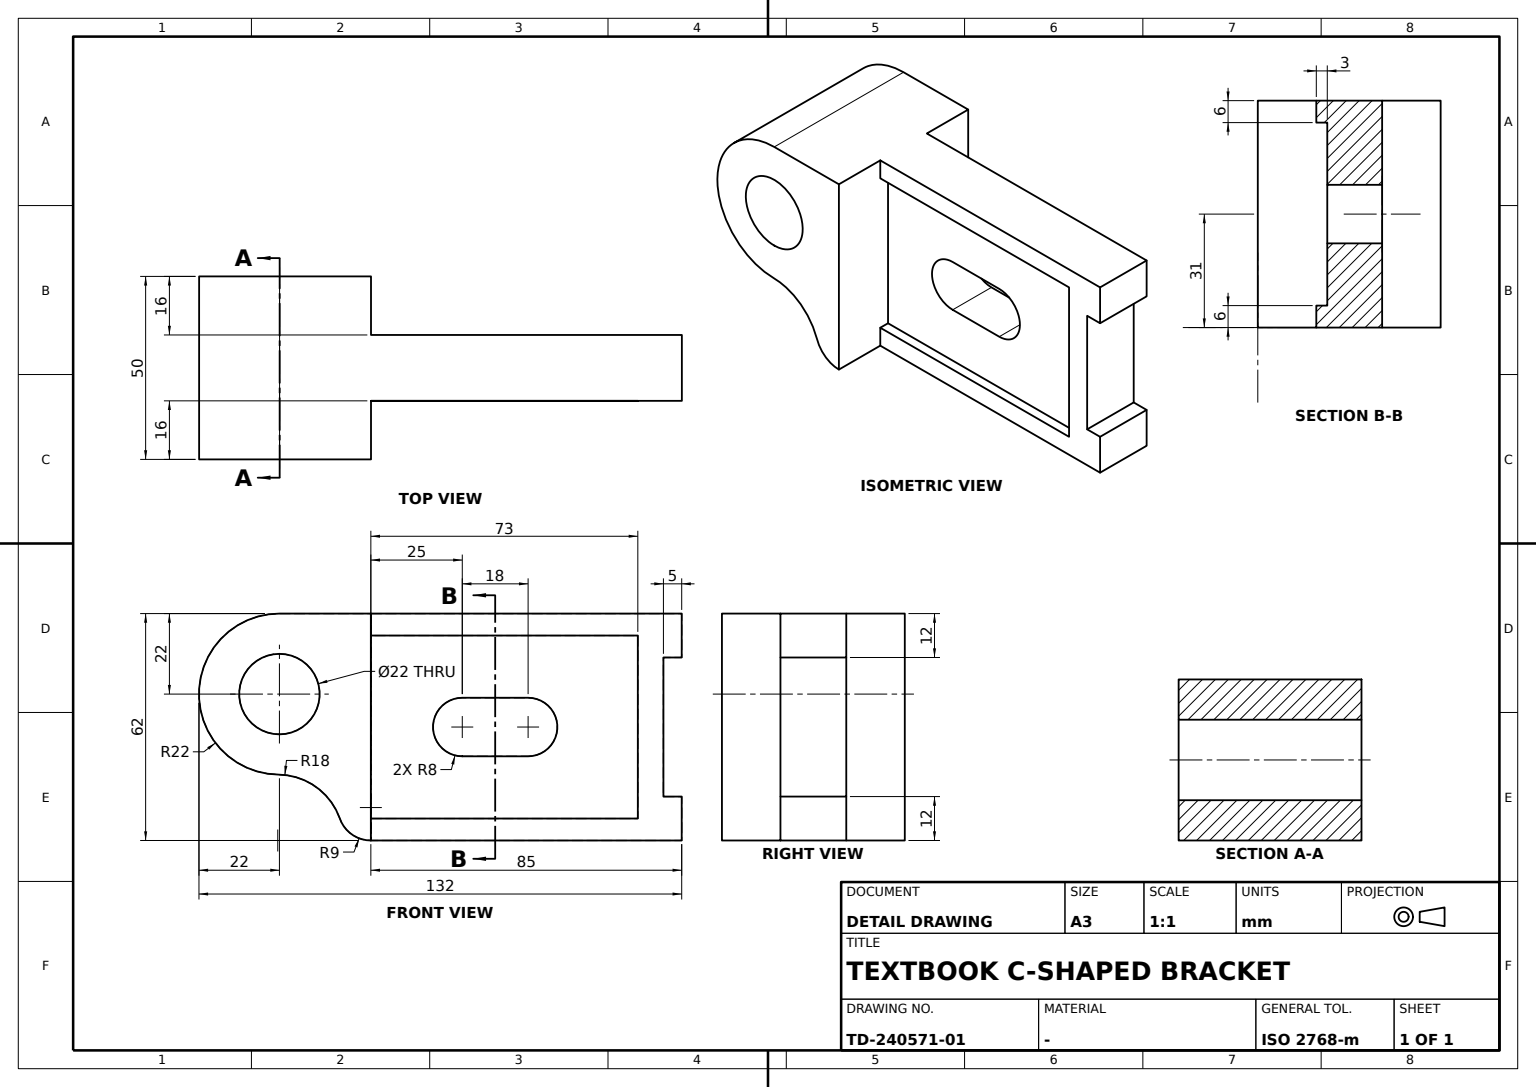
ISO-10303-21;
HEADER;
FILE_DESCRIPTION((''),'2;1');
FILE_NAME('','',(''),(''),'','','');
FILE_SCHEMA(('AUTOMOTIVE_DESIGN'));
ENDSEC;
DATA;
#1=APPLICATION_CONTEXT('');
#2=PRODUCT_CONTEXT('',#1,'mechanical');
#3=PRODUCT('','','',(#2));
#4=PRODUCT_DEFINITION_FORMATION('','',#3);
#5=PRODUCT_DEFINITION_CONTEXT('',#1,'design');
#6=PRODUCT_DEFINITION('','',#4,#5);
#7=PRODUCT_DEFINITION_SHAPE('','',#6);
#8=(LENGTH_UNIT()NAMED_UNIT(*)SI_UNIT(.MILLI.,.METRE.));
#9=(NAMED_UNIT(*)PLANE_ANGLE_UNIT()SI_UNIT($,.RADIAN.));
#10=(NAMED_UNIT(*)SI_UNIT($,.STERADIAN.)SOLID_ANGLE_UNIT());
#11=UNCERTAINTY_MEASURE_WITH_UNIT(LENGTH_MEASURE(0.005),#8,'distance_accuracy_value','');
#12=(GEOMETRIC_REPRESENTATION_CONTEXT(3)GLOBAL_UNCERTAINTY_ASSIGNED_CONTEXT((#11))GLOBAL_UNIT_ASSIGNED_CONTEXT((#8,#9,#10))REPRESENTATION_CONTEXT('',''));
#13=CARTESIAN_POINT('',(-9.,0.,-31.));
#14=VERTEX_POINT('',#13);
#15=CARTESIAN_POINT('',(-9.,0.,31.));
#16=VERTEX_POINT('',#15);
#17=CARTESIAN_POINT('',(-9.,0.,0.));
#18=DIRECTION('',(0.,0.,1.));
#19=VECTOR('',#18,1000.);
#20=LINE('',#17,#19);
#21=EDGE_CURVE('',#14,#16,#20,.T.);
#22=ORIENTED_EDGE('',*,*,#21,.F.);
#23=CARTESIAN_POINT('',(-25.,0.,-31.));
#24=VERTEX_POINT('',#23);
#25=DIRECTION('',(1.,0.,0.));
#26=VECTOR('',#25,1000.);
#27=LINE('',#23,#26);
#28=EDGE_CURVE('',#24,#14,#27,.T.);
#29=ORIENTED_EDGE('',*,*,#28,.F.);
#30=CARTESIAN_POINT('',(-25.,0.,31.));
#31=VERTEX_POINT('',#30);
#32=DIRECTION('',(0.,0.,-1.));
#33=VECTOR('',#32,1000.);
#34=LINE('',#23,#33);
#35=EDGE_CURVE('',#31,#24,#34,.T.);
#36=ORIENTED_EDGE('',*,*,#35,.F.);
#37=CARTESIAN_POINT('',(0.,0.,31.));
#38=LINE('',#37,#26);
#39=EDGE_CURVE('',#31,#16,#38,.T.);
#40=ORIENTED_EDGE('',*,*,#39,.T.);
#41=EDGE_LOOP('',(#22,#29,#36,#40));
#42=FACE_BOUND('',#41,.T.);
#43=CARTESIAN_POINT('',(0.,0.,-31.));
#44=DIRECTION('',(0.,1.,0.));
#45=AXIS2_PLACEMENT_3D('',#43,#44,#18);
#46=PLANE('',#45);
#47=ADVANCED_FACE('',(#42),#46,.T.);
#48=CARTESIAN_POINT('',(-25.,-25.,-2.));
#49=VERTEX_POINT('',#48);
#50=CARTESIAN_POINT('',(-25.,-25.,9.));
#51=AXIS2_PLACEMENT_3D('',#50,#25,#32);
#52=CIRCLE('',#51,11.);
#53=EDGE_CURVE('',#49,#49,#52,.T.);
#54=ORIENTED_EDGE('',*,*,#53,.F.);
#55=EDGE_LOOP('',(#54));
#56=FACE_BOUND('',#55,.T.);
#57=CARTESIAN_POINT('',(25.,-25.,-2.));
#58=VERTEX_POINT('',#57);
#59=CARTESIAN_POINT('',(25.,-25.,9.));
#60=AXIS2_PLACEMENT_3D('',#59,#25,#32);
#61=CIRCLE('',#60,11.);
#62=EDGE_CURVE('',#58,#58,#61,.T.);
#63=ORIENTED_EDGE('',*,*,#62,.T.);
#64=EDGE_LOOP('',(#63));
#65=FACE_BOUND('',#64,.T.);
#66=CARTESIAN_POINT('',(0.,-25.,9.));
#67=AXIS2_PLACEMENT_3D('',#66,#25,#44);
#68=CYLINDRICAL_SURFACE('',#67,11.);
#69=ADVANCED_FACE('',(#56,#65),#68,.F.);
#70=CARTESIAN_POINT('',(25.,-8.537319,-24.84854));
#71=VERTEX_POINT('',#70);
#72=CARTESIAN_POINT('',(25.,0.,-31.));
#73=VERTEX_POINT('',#72);
#74=CARTESIAN_POINT('',(25.,0.,-22.));
#75=AXIS2_PLACEMENT_3D('',#74,#25,#32);
#76=CIRCLE('',#75,9.);
#77=EDGE_CURVE('',#71,#73,#76,.T.);
#78=ORIENTED_EDGE('',*,*,#77,.T.);
#79=CARTESIAN_POINT('',(25.,0.,31.));
#80=VERTEX_POINT('',#79);
#81=LINE('',#72,#33);
#82=EDGE_CURVE('',#80,#73,#81,.T.);
#83=ORIENTED_EDGE('',*,*,#82,.F.);
#84=CARTESIAN_POINT('',(25.,-25.,31.));
#85=VERTEX_POINT('',#84);
#86=VECTOR('',#44,1000.);
#87=LINE('',#79,#86);
#88=EDGE_CURVE('',#85,#80,#87,.T.);
#89=ORIENTED_EDGE('',*,*,#88,.F.);
#90=CARTESIAN_POINT('',(25.,-25.24998,-12.99858));
#91=VERTEX_POINT('',#90);
#92=CIRCLE('',#60,22.);
#93=EDGE_CURVE('',#85,#91,#92,.T.);
#94=ORIENTED_EDGE('',*,*,#93,.T.);
#95=CARTESIAN_POINT('',(25.,-25.454509,-30.997418));
#96=AXIS2_PLACEMENT_3D('',#95,#25,#32);
#97=CIRCLE('',#96,18.);
#98=EDGE_CURVE('',#71,#91,#97,.T.);
#99=ORIENTED_EDGE('',*,*,#98,.F.);
#100=EDGE_LOOP('',(#78,#83,#89,#94,#99));
#101=FACE_BOUND('',#100,.T.);
#102=ORIENTED_EDGE('',*,*,#62,.F.);
#103=EDGE_LOOP('',(#102));
#104=FACE_BOUND('',#103,.T.);
#105=CARTESIAN_POINT('',(25.,0.,0.));
#106=AXIS2_PLACEMENT_3D('',#105,#25,#44);
#107=PLANE('',#106);
#108=ADVANCED_FACE('',(#101,#104),#107,.T.);
#109=CARTESIAN_POINT('',(6.,25.,-8.));
#110=VERTEX_POINT('',#109);
#111=CARTESIAN_POINT('',(6.,43.,-8.));
#112=VERTEX_POINT('',#111);
#113=LINE('',#109,#86);
#114=EDGE_CURVE('',#110,#112,#113,.T.);
#115=ORIENTED_EDGE('',*,*,#114,.T.);
#116=CARTESIAN_POINT('',(-9.,43.,-8.));
#117=VERTEX_POINT('',#116);
#118=CARTESIAN_POINT('',(-2.16,43.,-8.));
#119=LINE('',#118,#26);
#120=EDGE_CURVE('',#112,#117,#119,.F.);
#121=ORIENTED_EDGE('',*,*,#120,.T.);
#122=CARTESIAN_POINT('',(-9.,25.,-8.));
#123=VERTEX_POINT('',#122);
#124=LINE('',#122,#86);
#125=EDGE_CURVE('',#123,#117,#124,.T.);
#126=ORIENTED_EDGE('',*,*,#125,.F.);
#127=CARTESIAN_POINT('',(-2.16,25.,-8.));
#128=LINE('',#127,#26);
#129=EDGE_CURVE('',#110,#123,#128,.F.);
#130=ORIENTED_EDGE('',*,*,#129,.F.);
#131=EDGE_LOOP('',(#115,#121,#126,#130));
#132=FACE_BOUND('',#131,.T.);
#133=AXIS2_PLACEMENT_3D('',#109,#18,#44);
#134=PLANE('',#133);
#135=ADVANCED_FACE('',(#132),#134,.T.);
#136=CARTESIAN_POINT('',(6.,73.,25.));
#137=VERTEX_POINT('',#136);
#138=CARTESIAN_POINT('',(6.,73.,-25.));
#139=VERTEX_POINT('',#138);
#140=LINE('',#136,#33);
#141=EDGE_CURVE('',#137,#139,#140,.T.);
#142=ORIENTED_EDGE('',*,*,#141,.T.);
#143=CARTESIAN_POINT('',(9.,73.,-25.));
#144=VERTEX_POINT('',#143);
#145=DIRECTION('',(-1.,0.,0.));
#146=VECTOR('',#145,1000.);
#147=LINE('',#143,#146);
#148=EDGE_CURVE('',#144,#139,#147,.T.);
#149=ORIENTED_EDGE('',*,*,#148,.F.);
#150=CARTESIAN_POINT('',(9.,73.,25.));
#151=VERTEX_POINT('',#150);
#152=LINE('',#150,#33);
#153=EDGE_CURVE('',#151,#144,#152,.T.);
#154=ORIENTED_EDGE('',*,*,#153,.F.);
#155=LINE('',#150,#146);
#156=EDGE_CURVE('',#151,#137,#155,.T.);
#157=ORIENTED_EDGE('',*,*,#156,.T.);
#158=EDGE_LOOP('',(#142,#149,#154,#157));
#159=FACE_BOUND('',#158,.T.);
#160=AXIS2_PLACEMENT_3D('',#150,#44,#32);
#161=PLANE('',#160);
#162=ADVANCED_FACE('',(#159),#161,.F.);
#163=ORIENTED_EDGE('',*,*,#53,.T.);
#164=EDGE_LOOP('',(#163));
#165=FACE_BOUND('',#164,.T.);
#166=CARTESIAN_POINT('',(-25.,-8.537319,-24.84854));
#167=VERTEX_POINT('',#166);
#168=CARTESIAN_POINT('',(-25.,-25.24998,-12.99858));
#169=VERTEX_POINT('',#168);
#170=CARTESIAN_POINT('',(-25.,-25.454509,-30.997418));
#171=AXIS2_PLACEMENT_3D('',#170,#25,#32);
#172=CIRCLE('',#171,18.);
#173=EDGE_CURVE('',#167,#169,#172,.T.);
#174=ORIENTED_EDGE('',*,*,#173,.T.);
#175=CARTESIAN_POINT('',(-25.,-25.,31.));
#176=VERTEX_POINT('',#175);
#177=CIRCLE('',#51,22.);
#178=EDGE_CURVE('',#176,#169,#177,.T.);
#179=ORIENTED_EDGE('',*,*,#178,.F.);
#180=LINE('',#30,#86);
#181=EDGE_CURVE('',#176,#31,#180,.T.);
#182=ORIENTED_EDGE('',*,*,#181,.T.);
#183=ORIENTED_EDGE('',*,*,#35,.T.);
#184=CARTESIAN_POINT('',(-25.,0.,-22.));
#185=AXIS2_PLACEMENT_3D('',#184,#25,#32);
#186=CIRCLE('',#185,9.);
#187=EDGE_CURVE('',#167,#24,#186,.T.);
#188=ORIENTED_EDGE('',*,*,#187,.F.);
#189=EDGE_LOOP('',(#174,#179,#182,#183,#188));
#190=FACE_BOUND('',#189,.T.);
#191=CARTESIAN_POINT('',(-25.,0.,0.));
#192=AXIS2_PLACEMENT_3D('',#191,#25,#44);
#193=PLANE('',#192);
#194=ADVANCED_FACE('',(#165,#190),#193,.F.);
#195=LINE('',#166,#26);
#196=EDGE_CURVE('',#167,#71,#195,.T.);
#197=ORIENTED_EDGE('',*,*,#196,.T.);
#198=ORIENTED_EDGE('',*,*,#98,.T.);
#199=CARTESIAN_POINT('',(0.,-25.24998,-12.99858));
#200=LINE('',#199,#26);
#201=EDGE_CURVE('',#169,#91,#200,.T.);
#202=ORIENTED_EDGE('',*,*,#201,.F.);
#203=ORIENTED_EDGE('',*,*,#173,.F.);
#204=EDGE_LOOP('',(#197,#198,#202,#203));
#205=FACE_BOUND('',#204,.T.);
#206=CARTESIAN_POINT('',(0.,-25.454509,-30.997418));
#207=AXIS2_PLACEMENT_3D('',#206,#25,#44);
#208=CYLINDRICAL_SURFACE('',#207,18.);
#209=ADVANCED_FACE('',(#205),#208,.F.);
#210=CARTESIAN_POINT('',(6.,43.,8.));
#211=VERTEX_POINT('',#210);
#212=CARTESIAN_POINT('',(-9.,43.,8.));
#213=VERTEX_POINT('',#212);
#214=CARTESIAN_POINT('',(-2.16,43.,8.));
#215=LINE('',#214,#26);
#216=EDGE_CURVE('',#211,#213,#215,.F.);
#217=ORIENTED_EDGE('',*,*,#216,.T.);
#218=CARTESIAN_POINT('',(-9.,43.,0.));
#219=AXIS2_PLACEMENT_3D('',#218,#25,#32);
#220=CIRCLE('',#219,8.);
#221=EDGE_CURVE('',#117,#213,#220,.T.);
#222=ORIENTED_EDGE('',*,*,#221,.F.);
#223=ORIENTED_EDGE('',*,*,#120,.F.);
#224=CARTESIAN_POINT('',(6.,43.,0.));
#225=AXIS2_PLACEMENT_3D('',#224,#25,#32);
#226=CIRCLE('',#225,8.);
#227=EDGE_CURVE('',#112,#211,#226,.T.);
#228=ORIENTED_EDGE('',*,*,#227,.T.);
#229=EDGE_LOOP('',(#217,#222,#223,#228));
#230=FACE_BOUND('',#229,.T.);
#231=CARTESIAN_POINT('',(-2.16,43.,0.));
#232=AXIS2_PLACEMENT_3D('',#231,#25,#44);
#233=CYLINDRICAL_SURFACE('',#232,8.);
#234=ADVANCED_FACE('',(#230),#233,.F.);
#235=CARTESIAN_POINT('',(6.,25.,8.));
#236=VERTEX_POINT('',#235);
#237=CARTESIAN_POINT('',(-9.,25.,8.));
#238=VERTEX_POINT('',#237);
#239=CARTESIAN_POINT('',(-2.16,25.,8.));
#240=LINE('',#239,#26);
#241=EDGE_CURVE('',#236,#238,#240,.F.);
#242=ORIENTED_EDGE('',*,*,#241,.T.);
#243=LINE('',#237,#86);
#244=EDGE_CURVE('',#238,#213,#243,.T.);
#245=ORIENTED_EDGE('',*,*,#244,.T.);
#246=ORIENTED_EDGE('',*,*,#216,.F.);
#247=LINE('',#235,#86);
#248=EDGE_CURVE('',#236,#211,#247,.T.);
#249=ORIENTED_EDGE('',*,*,#248,.F.);
#250=EDGE_LOOP('',(#242,#245,#246,#249));
#251=FACE_BOUND('',#250,.T.);
#252=AXIS2_PLACEMENT_3D('',#235,#18,#44);
#253=PLANE('',#252);
#254=ADVANCED_FACE('',(#251),#253,.F.);
#255=CARTESIAN_POINT('',(-9.,80.,-19.));
#256=VERTEX_POINT('',#255);
#257=CARTESIAN_POINT('',(9.,80.,-19.));
#258=VERTEX_POINT('',#257);
#259=CARTESIAN_POINT('',(0.,80.,-19.));
#260=LINE('',#259,#26);
#261=EDGE_CURVE('',#256,#258,#260,.T.);
#262=ORIENTED_EDGE('',*,*,#261,.T.);
#263=CARTESIAN_POINT('',(9.,85.,-19.));
#264=VERTEX_POINT('',#263);
#265=CARTESIAN_POINT('',(9.,0.,-19.));
#266=LINE('',#265,#86);
#267=EDGE_CURVE('',#258,#264,#266,.T.);
#268=ORIENTED_EDGE('',*,*,#267,.T.);
#269=CARTESIAN_POINT('',(-9.,85.,-19.));
#270=VERTEX_POINT('',#269);
#271=CARTESIAN_POINT('',(0.,85.,-19.));
#272=LINE('',#271,#26);
#273=EDGE_CURVE('',#270,#264,#272,.T.);
#274=ORIENTED_EDGE('',*,*,#273,.F.);
#275=CARTESIAN_POINT('',(-9.,0.,-19.));
#276=LINE('',#275,#86);
#277=EDGE_CURVE('',#256,#270,#276,.T.);
#278=ORIENTED_EDGE('',*,*,#277,.F.);
#279=EDGE_LOOP('',(#262,#268,#274,#278));
#280=FACE_BOUND('',#279,.T.);
#281=AXIS2_PLACEMENT_3D('',#259,#32,#44);
#282=PLANE('',#281);
#283=ADVANCED_FACE('',(#280),#282,.F.);
#284=CARTESIAN_POINT('',(9.,0.,31.));
#285=VERTEX_POINT('',#284);
#286=EDGE_CURVE('',#285,#80,#38,.T.);
#287=ORIENTED_EDGE('',*,*,#286,.F.);
#288=CARTESIAN_POINT('',(9.,85.,31.));
#289=VERTEX_POINT('',#288);
#290=LINE('',#284,#86);
#291=EDGE_CURVE('',#285,#289,#290,.T.);
#292=ORIENTED_EDGE('',*,*,#291,.T.);
#293=CARTESIAN_POINT('',(-9.,85.,31.));
#294=VERTEX_POINT('',#293);
#295=CARTESIAN_POINT('',(0.,85.,31.));
#296=LINE('',#295,#26);
#297=EDGE_CURVE('',#294,#289,#296,.T.);
#298=ORIENTED_EDGE('',*,*,#297,.F.);
#299=LINE('',#15,#86);
#300=EDGE_CURVE('',#16,#294,#299,.T.);
#301=ORIENTED_EDGE('',*,*,#300,.F.);
#302=ORIENTED_EDGE('',*,*,#39,.F.);
#303=ORIENTED_EDGE('',*,*,#181,.F.);
#304=CARTESIAN_POINT('',(0.,-25.,31.));
#305=LINE('',#304,#26);
#306=EDGE_CURVE('',#176,#85,#305,.T.);
#307=ORIENTED_EDGE('',*,*,#306,.T.);
#308=ORIENTED_EDGE('',*,*,#88,.T.);
#309=EDGE_LOOP('',(#287,#292,#298,#301,#302,#303,#307,#308));
#310=FACE_BOUND('',#309,.T.);
#311=AXIS2_PLACEMENT_3D('',#37,#32,#44);
#312=PLANE('',#311);
#313=ADVANCED_FACE('',(#310),#312,.F.);
#314=ORIENTED_EDGE('',*,*,#241,.F.);
#315=CARTESIAN_POINT('',(6.,25.,0.));
#316=AXIS2_PLACEMENT_3D('',#315,#25,#32);
#317=CIRCLE('',#316,8.);
#318=EDGE_CURVE('',#236,#110,#317,.T.);
#319=ORIENTED_EDGE('',*,*,#318,.T.);
#320=ORIENTED_EDGE('',*,*,#129,.T.);
#321=CARTESIAN_POINT('',(-9.,25.,0.));
#322=AXIS2_PLACEMENT_3D('',#321,#25,#32);
#323=CIRCLE('',#322,8.);
#324=EDGE_CURVE('',#238,#123,#323,.T.);
#325=ORIENTED_EDGE('',*,*,#324,.F.);
#326=EDGE_LOOP('',(#314,#319,#320,#325));
#327=FACE_BOUND('',#326,.T.);
#328=CARTESIAN_POINT('',(-2.16,25.,0.));
#329=AXIS2_PLACEMENT_3D('',#328,#25,#44);
#330=CYLINDRICAL_SURFACE('',#329,8.);
#331=ADVANCED_FACE('',(#327),#330,.F.);
#332=ORIENTED_EDGE('',*,*,#297,.T.);
#333=CARTESIAN_POINT('',(9.,85.,19.));
#334=VERTEX_POINT('',#333);
#335=CARTESIAN_POINT('',(9.,85.,0.));
#336=LINE('',#335,#33);
#337=EDGE_CURVE('',#289,#334,#336,.T.);
#338=ORIENTED_EDGE('',*,*,#337,.T.);
#339=CARTESIAN_POINT('',(-9.,85.,19.));
#340=VERTEX_POINT('',#339);
#341=CARTESIAN_POINT('',(0.,85.,19.));
#342=LINE('',#341,#26);
#343=EDGE_CURVE('',#340,#334,#342,.T.);
#344=ORIENTED_EDGE('',*,*,#343,.F.);
#345=CARTESIAN_POINT('',(-9.,85.,0.));
#346=LINE('',#345,#33);
#347=EDGE_CURVE('',#294,#340,#346,.T.);
#348=ORIENTED_EDGE('',*,*,#347,.F.);
#349=EDGE_LOOP('',(#332,#338,#344,#348));
#350=FACE_BOUND('',#349,.T.);
#351=DIRECTION('',(0.,-1.,0.));
#352=AXIS2_PLACEMENT_3D('',#271,#351,#32);
#353=PLANE('',#352);
#354=ADVANCED_FACE('',(#350),#353,.F.);
#355=ORIENTED_EDGE('',*,*,#286,.T.);
#356=ORIENTED_EDGE('',*,*,#82,.T.);
#357=CARTESIAN_POINT('',(9.,0.,-31.));
#358=VERTEX_POINT('',#357);
#359=LINE('',#357,#26);
#360=EDGE_CURVE('',#358,#73,#359,.T.);
#361=ORIENTED_EDGE('',*,*,#360,.F.);
#362=CARTESIAN_POINT('',(9.,0.,-25.));
#363=VERTEX_POINT('',#362);
#364=CARTESIAN_POINT('',(9.,0.,0.));
#365=LINE('',#364,#19);
#366=EDGE_CURVE('',#358,#363,#365,.T.);
#367=ORIENTED_EDGE('',*,*,#366,.T.);
#368=CARTESIAN_POINT('',(6.,0.,-25.));
#369=VERTEX_POINT('',#368);
#370=CARTESIAN_POINT('',(0.,0.,-25.));
#371=LINE('',#370,#146);
#372=EDGE_CURVE('',#363,#369,#371,.T.);
#373=ORIENTED_EDGE('',*,*,#372,.T.);
#374=CARTESIAN_POINT('',(6.,0.,25.));
#375=VERTEX_POINT('',#374);
#376=CARTESIAN_POINT('',(6.,0.,0.));
#377=LINE('',#376,#19);
#378=EDGE_CURVE('',#369,#375,#377,.T.);
#379=ORIENTED_EDGE('',*,*,#378,.T.);
#380=CARTESIAN_POINT('',(9.,0.,25.));
#381=VERTEX_POINT('',#380);
#382=LINE('',#380,#146);
#383=EDGE_CURVE('',#381,#375,#382,.T.);
#384=ORIENTED_EDGE('',*,*,#383,.F.);
#385=EDGE_CURVE('',#381,#285,#365,.T.);
#386=ORIENTED_EDGE('',*,*,#385,.T.);
#387=EDGE_LOOP('',(#355,#356,#361,#367,#373,#379,#384,#386));
#388=FACE_BOUND('',#387,.T.);
#389=ADVANCED_FACE('',(#388),#46,.T.);
#390=CARTESIAN_POINT('',(9.,85.,-31.));
#391=VERTEX_POINT('',#390);
#392=EDGE_CURVE('',#264,#391,#336,.T.);
#393=ORIENTED_EDGE('',*,*,#392,.F.);
#394=ORIENTED_EDGE('',*,*,#267,.F.);
#395=CARTESIAN_POINT('',(9.,80.,19.));
#396=VERTEX_POINT('',#395);
#397=CARTESIAN_POINT('',(9.,80.,0.));
#398=LINE('',#397,#33);
#399=EDGE_CURVE('',#396,#258,#398,.T.);
#400=ORIENTED_EDGE('',*,*,#399,.F.);
#401=CARTESIAN_POINT('',(9.,0.,19.));
#402=VECTOR('',#351,1000.);
#403=LINE('',#401,#402);
#404=EDGE_CURVE('',#334,#396,#403,.T.);
#405=ORIENTED_EDGE('',*,*,#404,.F.);
#406=ORIENTED_EDGE('',*,*,#337,.F.);
#407=ORIENTED_EDGE('',*,*,#291,.F.);
#408=ORIENTED_EDGE('',*,*,#385,.F.);
#409=LINE('',#380,#86);
#410=EDGE_CURVE('',#381,#151,#409,.T.);
#411=ORIENTED_EDGE('',*,*,#410,.T.);
#412=ORIENTED_EDGE('',*,*,#153,.T.);
#413=LINE('',#362,#402);
#414=EDGE_CURVE('',#144,#363,#413,.T.);
#415=ORIENTED_EDGE('',*,*,#414,.T.);
#416=ORIENTED_EDGE('',*,*,#366,.F.);
#417=LINE('',#357,#402);
#418=EDGE_CURVE('',#391,#358,#417,.T.);
#419=ORIENTED_EDGE('',*,*,#418,.F.);
#420=EDGE_LOOP('',(#393,#394,#400,#405,#406,#407,#408,#411,#412,#415,#416,#419));
#421=FACE_BOUND('',#420,.T.);
#422=AXIS2_PLACEMENT_3D('',#364,#25,#44);
#423=PLANE('',#422);
#424=ADVANCED_FACE('',(#421),#423,.T.);
#425=ORIENTED_EDGE('',*,*,#372,.F.);
#426=ORIENTED_EDGE('',*,*,#414,.F.);
#427=ORIENTED_EDGE('',*,*,#148,.T.);
#428=LINE('',#368,#402);
#429=EDGE_CURVE('',#139,#369,#428,.T.);
#430=ORIENTED_EDGE('',*,*,#429,.T.);
#431=EDGE_LOOP('',(#425,#426,#427,#430));
#432=FACE_BOUND('',#431,.T.);
#433=AXIS2_PLACEMENT_3D('',#362,#32,#351);
#434=PLANE('',#433);
#435=ADVANCED_FACE('',(#432),#434,.F.);
#436=ORIENTED_EDGE('',*,*,#244,.F.);
#437=ORIENTED_EDGE('',*,*,#324,.T.);
#438=ORIENTED_EDGE('',*,*,#125,.T.);
#439=ORIENTED_EDGE('',*,*,#221,.T.);
#440=EDGE_LOOP('',(#436,#437,#438,#439));
#441=FACE_BOUND('',#440,.T.);
#442=CARTESIAN_POINT('',(-9.,85.,-31.));
#443=VERTEX_POINT('',#442);
#444=EDGE_CURVE('',#270,#443,#346,.T.);
#445=ORIENTED_EDGE('',*,*,#444,.T.);
#446=LINE('',#13,#402);
#447=EDGE_CURVE('',#443,#14,#446,.T.);
#448=ORIENTED_EDGE('',*,*,#447,.T.);
#449=ORIENTED_EDGE('',*,*,#21,.T.);
#450=ORIENTED_EDGE('',*,*,#300,.T.);
#451=ORIENTED_EDGE('',*,*,#347,.T.);
#452=CARTESIAN_POINT('',(-9.,80.,19.));
#453=VERTEX_POINT('',#452);
#454=CARTESIAN_POINT('',(-9.,0.,19.));
#455=LINE('',#454,#402);
#456=EDGE_CURVE('',#340,#453,#455,.T.);
#457=ORIENTED_EDGE('',*,*,#456,.T.);
#458=CARTESIAN_POINT('',(-9.,80.,0.));
#459=LINE('',#458,#33);
#460=EDGE_CURVE('',#453,#256,#459,.T.);
#461=ORIENTED_EDGE('',*,*,#460,.T.);
#462=ORIENTED_EDGE('',*,*,#277,.T.);
#463=EDGE_LOOP('',(#445,#448,#449,#450,#451,#457,#461,#462));
#464=FACE_BOUND('',#463,.T.);
#465=AXIS2_PLACEMENT_3D('',#17,#25,#44);
#466=PLANE('',#465);
#467=ADVANCED_FACE('',(#441,#464),#466,.F.);
#468=ORIENTED_EDGE('',*,*,#343,.T.);
#469=ORIENTED_EDGE('',*,*,#404,.T.);
#470=CARTESIAN_POINT('',(0.,80.,19.));
#471=LINE('',#470,#26);
#472=EDGE_CURVE('',#453,#396,#471,.T.);
#473=ORIENTED_EDGE('',*,*,#472,.F.);
#474=ORIENTED_EDGE('',*,*,#456,.F.);
#475=EDGE_LOOP('',(#468,#469,#473,#474));
#476=FACE_BOUND('',#475,.T.);
#477=AXIS2_PLACEMENT_3D('',#341,#18,#351);
#478=PLANE('',#477);
#479=ADVANCED_FACE('',(#476),#478,.F.);
#480=LINE('',#43,#26);
#481=EDGE_CURVE('',#14,#358,#480,.T.);
#482=ORIENTED_EDGE('',*,*,#481,.T.);
#483=ORIENTED_EDGE('',*,*,#360,.T.);
#484=ORIENTED_EDGE('',*,*,#77,.F.);
#485=ORIENTED_EDGE('',*,*,#196,.F.);
#486=ORIENTED_EDGE('',*,*,#187,.T.);
#487=ORIENTED_EDGE('',*,*,#28,.T.);
#488=EDGE_LOOP('',(#482,#483,#484,#485,#486,#487));
#489=FACE_BOUND('',#488,.T.);
#490=CARTESIAN_POINT('',(0.,0.,-22.));
#491=AXIS2_PLACEMENT_3D('',#490,#25,#44);
#492=CYLINDRICAL_SURFACE('',#491,9.);
#493=ADVANCED_FACE('',(#489),#492,.T.);
#494=ORIENTED_EDGE('',*,*,#418,.T.);
#495=ORIENTED_EDGE('',*,*,#481,.F.);
#496=ORIENTED_EDGE('',*,*,#447,.F.);
#497=CARTESIAN_POINT('',(0.,85.,-31.));
#498=LINE('',#497,#26);
#499=EDGE_CURVE('',#443,#391,#498,.T.);
#500=ORIENTED_EDGE('',*,*,#499,.T.);
#501=EDGE_LOOP('',(#494,#495,#496,#500));
#502=FACE_BOUND('',#501,.T.);
#503=AXIS2_PLACEMENT_3D('',#497,#18,#351);
#504=PLANE('',#503);
#505=ADVANCED_FACE('',(#502),#504,.F.);
#506=ORIENTED_EDGE('',*,*,#460,.F.);
#507=ORIENTED_EDGE('',*,*,#472,.T.);
#508=ORIENTED_EDGE('',*,*,#399,.T.);
#509=ORIENTED_EDGE('',*,*,#261,.F.);
#510=EDGE_LOOP('',(#506,#507,#508,#509));
#511=FACE_BOUND('',#510,.T.);
#512=AXIS2_PLACEMENT_3D('',#470,#351,#32);
#513=PLANE('',#512);
#514=ADVANCED_FACE('',(#511),#513,.F.);
#515=ORIENTED_EDGE('',*,*,#141,.F.);
#516=LINE('',#374,#86);
#517=EDGE_CURVE('',#375,#137,#516,.T.);
#518=ORIENTED_EDGE('',*,*,#517,.F.);
#519=ORIENTED_EDGE('',*,*,#378,.F.);
#520=ORIENTED_EDGE('',*,*,#429,.F.);
#521=EDGE_LOOP('',(#515,#518,#519,#520));
#522=FACE_BOUND('',#521,.T.);
#523=ORIENTED_EDGE('',*,*,#114,.F.);
#524=ORIENTED_EDGE('',*,*,#318,.F.);
#525=ORIENTED_EDGE('',*,*,#248,.T.);
#526=ORIENTED_EDGE('',*,*,#227,.F.);
#527=EDGE_LOOP('',(#523,#524,#525,#526));
#528=FACE_BOUND('',#527,.T.);
#529=AXIS2_PLACEMENT_3D('',#376,#25,#44);
#530=PLANE('',#529);
#531=ADVANCED_FACE('',(#522,#528),#530,.T.);
#532=ORIENTED_EDGE('',*,*,#178,.T.);
#533=ORIENTED_EDGE('',*,*,#201,.T.);
#534=ORIENTED_EDGE('',*,*,#93,.F.);
#535=ORIENTED_EDGE('',*,*,#306,.F.);
#536=EDGE_LOOP('',(#532,#533,#534,#535));
#537=FACE_BOUND('',#536,.T.);
#538=CYLINDRICAL_SURFACE('',#67,22.);
#539=ADVANCED_FACE('',(#537),#538,.T.);
#540=ORIENTED_EDGE('',*,*,#383,.T.);
#541=ORIENTED_EDGE('',*,*,#517,.T.);
#542=ORIENTED_EDGE('',*,*,#156,.F.);
#543=ORIENTED_EDGE('',*,*,#410,.F.);
#544=EDGE_LOOP('',(#540,#541,#542,#543));
#545=FACE_BOUND('',#544,.T.);
#546=AXIS2_PLACEMENT_3D('',#380,#18,#44);
#547=PLANE('',#546);
#548=ADVANCED_FACE('',(#545),#547,.F.);
#549=ORIENTED_EDGE('',*,*,#392,.T.);
#550=ORIENTED_EDGE('',*,*,#499,.F.);
#551=ORIENTED_EDGE('',*,*,#444,.F.);
#552=ORIENTED_EDGE('',*,*,#273,.T.);
#553=EDGE_LOOP('',(#549,#550,#551,#552));
#554=FACE_BOUND('',#553,.T.);
#555=ADVANCED_FACE('',(#554),#353,.F.);
#556=CLOSED_SHELL('',(#47,#69,#108,#135,#162,#194,#209,#234,#254,#283,#313,#331,#354,#389,#424,#435,#467,#479,#493,#505,#514,#531,#539,#548,#555));
#557=MANIFOLD_SOLID_BREP('',#556);
#558=ADVANCED_BREP_SHAPE_REPRESENTATION('',(#557),#12);
#559=SHAPE_DEFINITION_REPRESENTATION(#7,#558);
ENDSEC;
END-ISO-10303-21;
